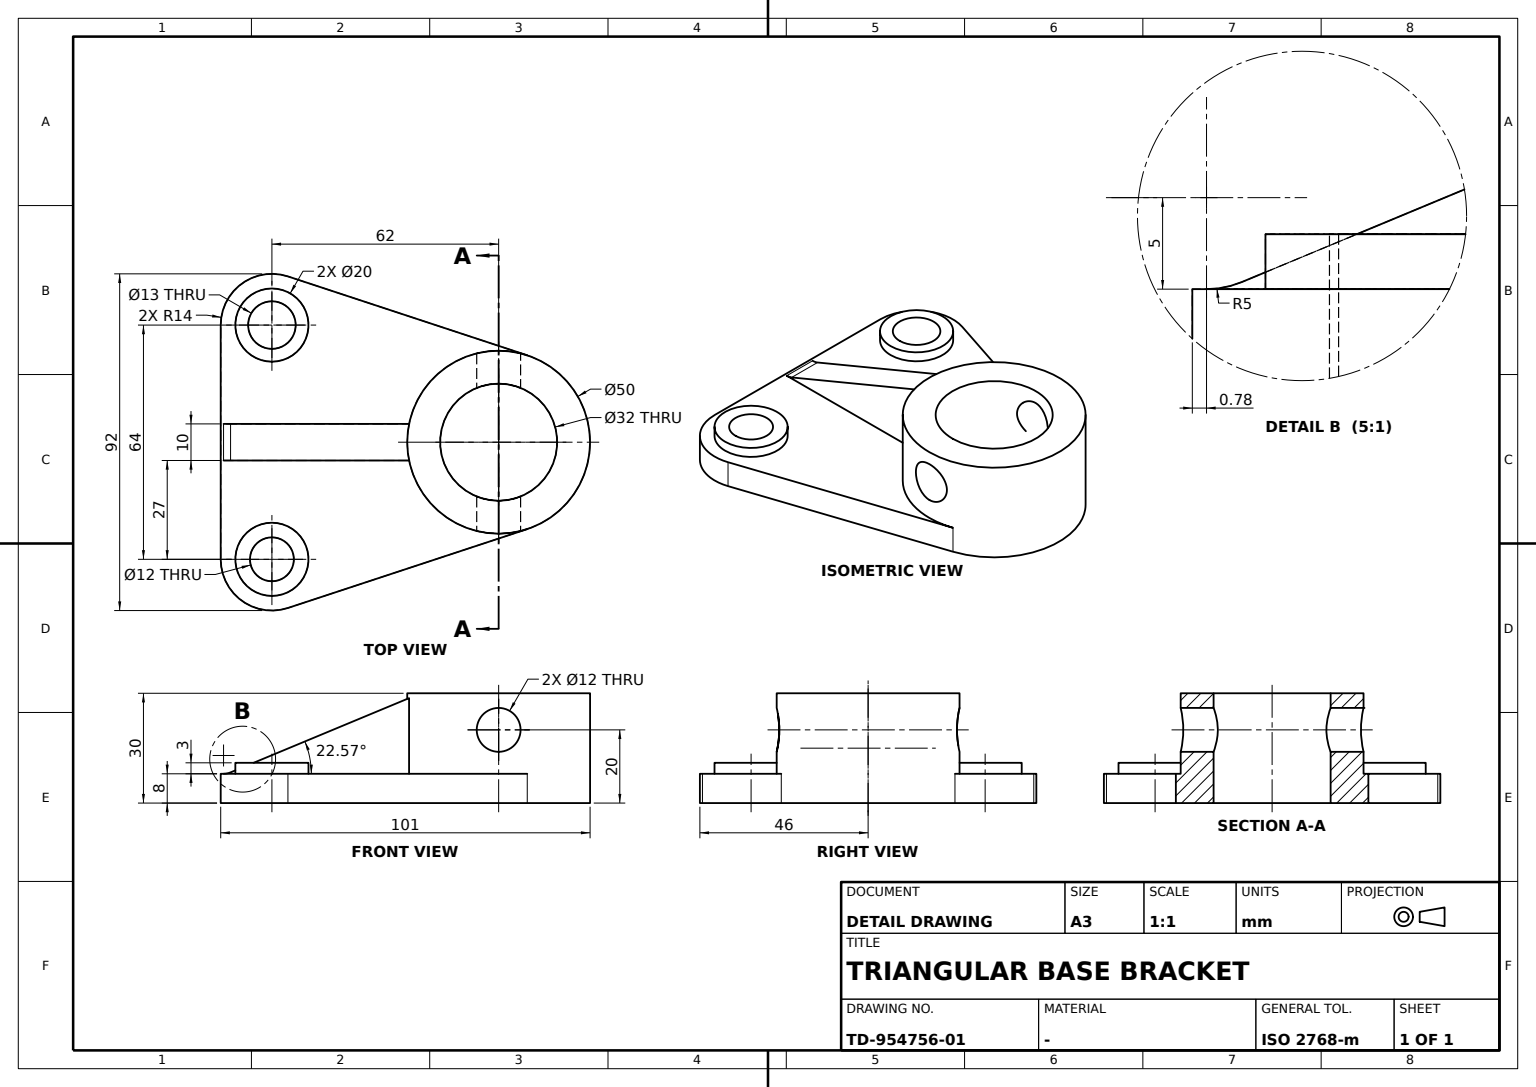
ISO-10303-21;
HEADER;
FILE_DESCRIPTION((''),'2;1');
FILE_NAME('','',(''),(''),'','','');
FILE_SCHEMA(('AUTOMOTIVE_DESIGN'));
ENDSEC;
DATA;
#1=APPLICATION_CONTEXT('');
#2=PRODUCT_CONTEXT('',#1,'mechanical');
#3=PRODUCT('','','',(#2));
#4=PRODUCT_DEFINITION_FORMATION('','',#3);
#5=PRODUCT_DEFINITION_CONTEXT('',#1,'design');
#6=PRODUCT_DEFINITION('','',#4,#5);
#7=PRODUCT_DEFINITION_SHAPE('','',#6);
#8=(LENGTH_UNIT()NAMED_UNIT(*)SI_UNIT(.MILLI.,.METRE.));
#9=(NAMED_UNIT(*)PLANE_ANGLE_UNIT()SI_UNIT($,.RADIAN.));
#10=(NAMED_UNIT(*)SI_UNIT($,.STERADIAN.)SOLID_ANGLE_UNIT());
#11=UNCERTAINTY_MEASURE_WITH_UNIT(LENGTH_MEASURE(0.005),#8,'distance_accuracy_value','');
#12=(GEOMETRIC_REPRESENTATION_CONTEXT(3)GLOBAL_UNCERTAINTY_ASSIGNED_CONTEXT((#11))GLOBAL_UNIT_ASSIGNED_CONTEXT((#8,#9,#10))REPRESENTATION_CONTEXT('',''));
#13=CARTESIAN_POINT('',(5.,-24.494897,8.));
#14=VERTEX_POINT('',#13);
#15=CARTESIAN_POINT('',(5.,-24.494897,28.67148));
#16=VERTEX_POINT('',#15);
#17=DIRECTION('',(0.,0.,1.));
#18=VECTOR('',#17,1000.);
#19=LINE('',#13,#18);
#20=EDGE_CURVE('',#14,#16,#19,.T.);
#21=ORIENTED_EDGE('',*,*,#20,.T.);
#22=CARTESIAN_POINT('',(5.,-73.303678,8.382988));
#23=VERTEX_POINT('',#22);
#24=CARTESIAN_POINT('',(5.,-76.,7.2622));
#25=DIRECTION('',(0.,0.923402354,0.383833418));
#26=VECTOR('',#25,1000.);
#27=LINE('',#24,#26);
#28=EDGE_CURVE('',#23,#16,#27,.T.);
#29=ORIENTED_EDGE('',*,*,#28,.F.);
#30=CARTESIAN_POINT('',(5.,-75.222845,8.));
#31=VERTEX_POINT('',#30);
#32=CARTESIAN_POINT('',(5.,-75.222845,13.));
#33=DIRECTION('',(1.,0.,0.));
#34=DIRECTION('',(0.,0.,-1.));
#35=AXIS2_PLACEMENT_3D('',#32,#33,#34);
#36=CIRCLE('',#35,5.);
#37=EDGE_CURVE('',#31,#23,#36,.T.);
#38=ORIENTED_EDGE('',*,*,#37,.F.);
#39=CARTESIAN_POINT('',(5.,0.,8.));
#40=DIRECTION('',(0.,-1.,0.));
#41=VECTOR('',#40,1000.);
#42=LINE('',#39,#41);
#43=EDGE_CURVE('',#14,#31,#42,.T.);
#44=ORIENTED_EDGE('',*,*,#43,.F.);
#45=EDGE_LOOP('',(#21,#29,#38,#44));
#46=FACE_BOUND('',#45,.T.);
#47=CARTESIAN_POINT('',(5.,0.,0.));
#48=DIRECTION('',(0.,1.,0.));
#49=AXIS2_PLACEMENT_3D('',#47,#33,#48);
#50=PLANE('',#49);
#51=ADVANCED_FACE('',(#46),#50,.T.);
#52=CARTESIAN_POINT('',(-25.5,-62.,0.));
#53=VERTEX_POINT('',#52);
#54=CARTESIAN_POINT('',(-32.,-62.,0.));
#55=AXIS2_PLACEMENT_3D('',#54,#17,#33);
#56=CIRCLE('',#55,6.5);
#57=EDGE_CURVE('',#53,#53,#56,.T.);
#58=ORIENTED_EDGE('',*,*,#57,.T.);
#59=EDGE_LOOP('',(#58));
#60=FACE_BOUND('',#59,.T.);
#61=CARTESIAN_POINT('',(16.,0.,0.));
#62=VERTEX_POINT('',#61);
#63=CARTESIAN_POINT('',(0.,0.,0.));
#64=AXIS2_PLACEMENT_3D('',#63,#17,#33);
#65=CIRCLE('',#64,16.);
#66=EDGE_CURVE('',#62,#62,#65,.T.);
#67=ORIENTED_EDGE('',*,*,#66,.T.);
#68=EDGE_LOOP('',(#67));
#69=FACE_BOUND('',#68,.T.);
#70=CARTESIAN_POINT('',(-45.297428,-57.620683,0.));
#71=VERTEX_POINT('',#70);
#72=CARTESIAN_POINT('',(-32.,-76.,0.));
#73=VERTEX_POINT('',#72);
#74=CIRCLE('',#55,14.);
#75=EDGE_CURVE('',#71,#73,#74,.T.);
#76=ORIENTED_EDGE('',*,*,#75,.F.);
#77=CARTESIAN_POINT('',(-23.745406,7.82021,0.));
#78=VERTEX_POINT('',#77);
#79=DIRECTION('',(-0.312808388,-0.949816252,0.));
#80=VECTOR('',#79,1000.);
#81=LINE('',#77,#80);
#82=EDGE_CURVE('',#78,#71,#81,.T.);
#83=ORIENTED_EDGE('',*,*,#82,.F.);
#84=CARTESIAN_POINT('',(23.745406,7.82021,0.));
#85=VERTEX_POINT('',#84);
#86=CIRCLE('',#64,25.);
#87=EDGE_CURVE('',#85,#78,#86,.T.);
#88=ORIENTED_EDGE('',*,*,#87,.F.);
#89=CARTESIAN_POINT('',(45.297428,-57.620683,0.));
#90=VERTEX_POINT('',#89);
#91=DIRECTION('',(0.312808388,-0.949816252,0.));
#92=VECTOR('',#91,1000.);
#93=LINE('',#84,#92);
#94=EDGE_CURVE('',#85,#90,#93,.T.);
#95=ORIENTED_EDGE('',*,*,#94,.T.);
#96=CARTESIAN_POINT('',(32.,-76.,0.));
#97=VERTEX_POINT('',#96);
#98=CARTESIAN_POINT('',(32.,-62.,0.));
#99=AXIS2_PLACEMENT_3D('',#98,#17,#33);
#100=CIRCLE('',#99,14.);
#101=EDGE_CURVE('',#97,#90,#100,.T.);
#102=ORIENTED_EDGE('',*,*,#101,.F.);
#103=CARTESIAN_POINT('',(0.,-76.,0.));
#104=VECTOR('',#33,1000.);
#105=LINE('',#103,#104);
#106=EDGE_CURVE('',#73,#97,#105,.T.);
#107=ORIENTED_EDGE('',*,*,#106,.F.);
#108=EDGE_LOOP('',(#76,#83,#88,#95,#102,#107));
#109=FACE_BOUND('',#108,.T.);
#110=CARTESIAN_POINT('',(38.,-62.,0.));
#111=VERTEX_POINT('',#110);
#112=CIRCLE('',#99,6.);
#113=EDGE_CURVE('',#111,#111,#112,.T.);
#114=ORIENTED_EDGE('',*,*,#113,.T.);
#115=EDGE_LOOP('',(#114));
#116=FACE_BOUND('',#115,.T.);
#117=PLANE('',#64);
#118=ADVANCED_FACE('',(#60,#69,#109,#116),#117,.F.);
#119=CARTESIAN_POINT('',(-45.297428,-57.620683,8.));
#120=VERTEX_POINT('',#119);
#121=CARTESIAN_POINT('',(-45.297428,-57.620683,4.));
#122=LINE('',#121,#18);
#123=EDGE_CURVE('',#71,#120,#122,.T.);
#124=ORIENTED_EDGE('',*,*,#123,.F.);
#125=ORIENTED_EDGE('',*,*,#75,.T.);
#126=CARTESIAN_POINT('',(-32.,-76.,8.));
#127=VERTEX_POINT('',#126);
#128=CARTESIAN_POINT('',(-32.,-76.,4.));
#129=LINE('',#128,#18);
#130=EDGE_CURVE('',#73,#127,#129,.T.);
#131=ORIENTED_EDGE('',*,*,#130,.T.);
#132=CARTESIAN_POINT('',(-32.,-62.,8.));
#133=AXIS2_PLACEMENT_3D('',#132,#17,#33);
#134=CIRCLE('',#133,14.);
#135=EDGE_CURVE('',#120,#127,#134,.T.);
#136=ORIENTED_EDGE('',*,*,#135,.F.);
#137=EDGE_LOOP('',(#124,#125,#131,#136));
#138=FACE_BOUND('',#137,.T.);
#139=CARTESIAN_POINT('',(-32.,-62.,4.));
#140=AXIS2_PLACEMENT_3D('',#139,#17,#33);
#141=CYLINDRICAL_SURFACE('',#140,14.);
#142=ADVANCED_FACE('',(#138),#141,.T.);
#143=CARTESIAN_POINT('',(-22.,-62.,8.));
#144=VERTEX_POINT('',#143);
#145=CIRCLE('',#133,10.);
#146=EDGE_CURVE('',#144,#144,#145,.T.);
#147=ORIENTED_EDGE('',*,*,#146,.T.);
#148=EDGE_LOOP('',(#147));
#149=FACE_BOUND('',#148,.T.);
#150=CARTESIAN_POINT('',(-22.,-62.,11.));
#151=VERTEX_POINT('',#150);
#152=CARTESIAN_POINT('',(-32.,-62.,11.));
#153=AXIS2_PLACEMENT_3D('',#152,#17,#33);
#154=CIRCLE('',#153,10.);
#155=EDGE_CURVE('',#151,#151,#154,.T.);
#156=ORIENTED_EDGE('',*,*,#155,.F.);
#157=EDGE_LOOP('',(#156));
#158=FACE_BOUND('',#157,.T.);
#159=CARTESIAN_POINT('',(-32.,-62.,9.5));
#160=AXIS2_PLACEMENT_3D('',#159,#17,#33);
#161=CYLINDRICAL_SURFACE('',#160,10.);
#162=ADVANCED_FACE('',(#149,#158),#161,.T.);
#163=CARTESIAN_POINT('',(14.832397,-6.,20.));
#164=VERTEX_POINT('',#163);
#165=CARTESIAN_POINT('',(15.438638,-4.702504,15.296631));
#166=CARTESIAN_POINT('',(14.529476,-6.648414,20.000931));
#167=CARTESIAN_POINT('',(15.437841,-4.703839,24.699646));
#168=CARTESIAN_POINT('',(16.281291,0.002975,26.651377));
#169=CARTESIAN_POINT('',(15.436993,4.705057,24.694845));
#170=CARTESIAN_POINT('',(14.529843,6.648585,20.009134));
#171=CARTESIAN_POINT('',(15.43802,4.700591,15.296493));
#172=CARTESIAN_POINT('',(16.280835,0.007567,13.351722));
#173=B_SPLINE_CURVE_WITH_KNOTS('',3,(#165,#166,#167,#168,#169,#170,#171,#172,#165,#166,#167),.UNSPECIFIED.,.T.,.F.,(1,1,1,1,1,1,1,1,1,1,1,1,1,1,1),(-0.014193849,-0.009462566,-0.004731283,0.,0.004731283,0.009462566,0.014193849,0.018925132,0.023656415,0.028387698,0.033118981,0.037850264,0.042581547,0.04731283,0.052044113),.UNSPECIFIED.);
#174=EDGE_CURVE('',#164,#164,#173,.T.);
#175=ORIENTED_EDGE('',*,*,#174,.T.);
#176=EDGE_LOOP('',(#175));
#177=FACE_BOUND('',#176,.T.);
#178=CARTESIAN_POINT('',(25.,0.,14.));
#179=VERTEX_POINT('',#178);
#180=CARTESIAN_POINT('',(24.640168,-4.700584,24.702732));
#181=CARTESIAN_POINT('',(24.083983,-6.649013,19.99808));
#182=CARTESIAN_POINT('',(24.639835,-4.703363,15.300168));
#183=CARTESIAN_POINT('',(25.179986,0.001317,13.350708));
#184=CARTESIAN_POINT('',(24.640221,4.700485,15.297001));
#185=CARTESIAN_POINT('',(24.083956,6.649063,20.00192));
#186=CARTESIAN_POINT('',(24.639887,4.703263,24.7001));
#187=CARTESIAN_POINT('',(25.179986,-0.002041,26.649292));
#188=B_SPLINE_CURVE_WITH_KNOTS('',3,(#180,#181,#182,#183,#184,#185,#186,#187,#180,#181,#182),.UNSPECIFIED.,.T.,.F.,(1,1,1,1,1,1,1,1,1,1,1,1,1,1,1),(0.004704535,0.009408284,0.014112033,0.018815782,0.023519531,0.02822328,0.032927029,0.037630779,0.042334528,0.047038277,0.051742026,0.056445775,0.061149524,0.065853273,0.070557022),.UNSPECIFIED.);
#189=EDGE_CURVE('',#179,#179,#188,.T.);
#190=ORIENTED_EDGE('',*,*,#189,.T.);
#191=EDGE_LOOP('',(#190));
#192=FACE_BOUND('',#191,.T.);
#193=CARTESIAN_POINT('',(23.66,0.,20.));
#194=AXIS2_PLACEMENT_3D('',#193,#33,#48);
#195=CYLINDRICAL_SURFACE('',#194,6.);
#196=ADVANCED_FACE('',(#177,#192),#195,.F.);
#197=CARTESIAN_POINT('',(-5.,-73.303678,8.382988));
#198=VERTEX_POINT('',#197);
#199=CARTESIAN_POINT('',(0.,-73.303678,8.382988));
#200=LINE('',#199,#104);
#201=EDGE_CURVE('',#198,#23,#200,.T.);
#202=ORIENTED_EDGE('',*,*,#201,.F.);
#203=CARTESIAN_POINT('',(-5.,-75.222845,8.));
#204=VERTEX_POINT('',#203);
#205=CARTESIAN_POINT('',(-5.,-75.222845,13.));
#206=AXIS2_PLACEMENT_3D('',#205,#33,#34);
#207=CIRCLE('',#206,5.);
#208=EDGE_CURVE('',#204,#198,#207,.T.);
#209=ORIENTED_EDGE('',*,*,#208,.F.);
#210=CARTESIAN_POINT('',(0.,-75.222845,8.));
#211=LINE('',#210,#104);
#212=EDGE_CURVE('',#204,#31,#211,.T.);
#213=ORIENTED_EDGE('',*,*,#212,.T.);
#214=ORIENTED_EDGE('',*,*,#37,.T.);
#215=EDGE_LOOP('',(#202,#209,#213,#214));
#216=FACE_BOUND('',#215,.T.);
#217=CARTESIAN_POINT('',(0.,-75.222845,13.));
#218=DIRECTION('',(0.,0.383833418,-0.923402354));
#219=AXIS2_PLACEMENT_3D('',#217,#33,#218);
#220=CYLINDRICAL_SURFACE('',#219,5.);
#221=ADVANCED_FACE('',(#216),#220,.F.);
#222=CARTESIAN_POINT('',(42.,-62.,8.));
#223=VERTEX_POINT('',#222);
#224=CARTESIAN_POINT('',(32.,-62.,8.));
#225=AXIS2_PLACEMENT_3D('',#224,#17,#33);
#226=CIRCLE('',#225,10.);
#227=EDGE_CURVE('',#223,#223,#226,.T.);
#228=ORIENTED_EDGE('',*,*,#227,.T.);
#229=EDGE_LOOP('',(#228));
#230=FACE_BOUND('',#229,.T.);
#231=CARTESIAN_POINT('',(42.,-62.,11.));
#232=VERTEX_POINT('',#231);
#233=CARTESIAN_POINT('',(32.,-62.,11.));
#234=AXIS2_PLACEMENT_3D('',#233,#17,#33);
#235=CIRCLE('',#234,10.);
#236=EDGE_CURVE('',#232,#232,#235,.T.);
#237=ORIENTED_EDGE('',*,*,#236,.F.);
#238=EDGE_LOOP('',(#237));
#239=FACE_BOUND('',#238,.T.);
#240=CARTESIAN_POINT('',(32.,-62.,9.5));
#241=AXIS2_PLACEMENT_3D('',#240,#17,#33);
#242=CYLINDRICAL_SURFACE('',#241,10.);
#243=ADVANCED_FACE('',(#230,#239),#242,.T.);
#244=CARTESIAN_POINT('',(32.,-76.,8.));
#245=VERTEX_POINT('',#244);
#246=CARTESIAN_POINT('',(45.297428,-57.620683,8.));
#247=VERTEX_POINT('',#246);
#248=CIRCLE('',#225,14.);
#249=EDGE_CURVE('',#245,#247,#248,.T.);
#250=ORIENTED_EDGE('',*,*,#249,.F.);
#251=CARTESIAN_POINT('',(32.,-76.,4.));
#252=LINE('',#251,#18);
#253=EDGE_CURVE('',#97,#245,#252,.T.);
#254=ORIENTED_EDGE('',*,*,#253,.F.);
#255=ORIENTED_EDGE('',*,*,#101,.T.);
#256=CARTESIAN_POINT('',(45.297428,-57.620683,4.));
#257=LINE('',#256,#18);
#258=EDGE_CURVE('',#90,#247,#257,.T.);
#259=ORIENTED_EDGE('',*,*,#258,.T.);
#260=EDGE_LOOP('',(#250,#254,#255,#259));
#261=FACE_BOUND('',#260,.T.);
#262=CARTESIAN_POINT('',(32.,-62.,4.));
#263=AXIS2_PLACEMENT_3D('',#262,#17,#33);
#264=CYLINDRICAL_SURFACE('',#263,14.);
#265=ADVANCED_FACE('',(#261),#264,.T.);
#266=CARTESIAN_POINT('',(-25.5,-62.,11.));
#267=VERTEX_POINT('',#266);
#268=CIRCLE('',#153,6.5);
#269=EDGE_CURVE('',#267,#267,#268,.T.);
#270=ORIENTED_EDGE('',*,*,#269,.F.);
#271=EDGE_LOOP('',(#270));
#272=FACE_BOUND('',#271,.T.);
#273=ORIENTED_EDGE('',*,*,#155,.T.);
#274=EDGE_LOOP('',(#273));
#275=FACE_BOUND('',#274,.T.);
#276=CARTESIAN_POINT('',(0.,0.,11.));
#277=AXIS2_PLACEMENT_3D('',#276,#17,#33);
#278=PLANE('',#277);
#279=ADVANCED_FACE('',(#272,#275),#278,.T.);
#280=ORIENTED_EDGE('',*,*,#227,.F.);
#281=EDGE_LOOP('',(#280));
#282=FACE_BOUND('',#281,.T.);
#283=ORIENTED_EDGE('',*,*,#43,.T.);
#284=ORIENTED_EDGE('',*,*,#212,.F.);
#285=CARTESIAN_POINT('',(-5.,-24.494897,8.));
#286=VERTEX_POINT('',#285);
#287=CARTESIAN_POINT('',(-5.,0.,8.));
#288=LINE('',#287,#41);
#289=EDGE_CURVE('',#286,#204,#288,.T.);
#290=ORIENTED_EDGE('',*,*,#289,.F.);
#291=CARTESIAN_POINT('',(-23.745406,7.82021,8.));
#292=VERTEX_POINT('',#291);
#293=CARTESIAN_POINT('',(0.,0.,8.));
#294=AXIS2_PLACEMENT_3D('',#293,#17,#33);
#295=CIRCLE('',#294,25.);
#296=EDGE_CURVE('',#292,#286,#295,.T.);
#297=ORIENTED_EDGE('',*,*,#296,.F.);
#298=LINE('',#291,#80);
#299=EDGE_CURVE('',#292,#120,#298,.T.);
#300=ORIENTED_EDGE('',*,*,#299,.T.);
#301=ORIENTED_EDGE('',*,*,#135,.T.);
#302=CARTESIAN_POINT('',(0.,-76.,8.));
#303=LINE('',#302,#104);
#304=EDGE_CURVE('',#127,#245,#303,.T.);
#305=ORIENTED_EDGE('',*,*,#304,.T.);
#306=ORIENTED_EDGE('',*,*,#249,.T.);
#307=CARTESIAN_POINT('',(23.745406,7.82021,8.));
#308=VERTEX_POINT('',#307);
#309=LINE('',#307,#92);
#310=EDGE_CURVE('',#308,#247,#309,.T.);
#311=ORIENTED_EDGE('',*,*,#310,.F.);
#312=EDGE_CURVE('',#14,#308,#295,.T.);
#313=ORIENTED_EDGE('',*,*,#312,.F.);
#314=EDGE_LOOP('',(#283,#284,#290,#297,#300,#301,#305,#306,#311,#313));
#315=FACE_BOUND('',#314,.T.);
#316=ORIENTED_EDGE('',*,*,#146,.F.);
#317=EDGE_LOOP('',(#316));
#318=FACE_BOUND('',#317,.T.);
#319=PLANE('',#294);
#320=ADVANCED_FACE('',(#282,#315,#318),#319,.T.);
#321=CARTESIAN_POINT('',(-14.832397,6.,20.));
#322=VERTEX_POINT('',#321);
#323=CARTESIAN_POINT('',(-15.43811,-4.702049,24.701313));
#324=CARTESIAN_POINT('',(-14.529709,-6.648345,19.999768));
#325=CARTESIAN_POINT('',(-15.437434,-4.704571,15.301256));
#326=CARTESIAN_POINT('',(-16.281119,0.000146,13.350008));
#327=CARTESIAN_POINT('',(-15.438088,4.702119,15.298712));
#328=CARTESIAN_POINT('',(-14.529709,6.648345,20.000424));
#329=CARTESIAN_POINT('',(-15.437456,4.704501,24.69877));
#330=CARTESIAN_POINT('',(-16.281108,-0.000146,26.649979));
#331=B_SPLINE_CURVE_WITH_KNOTS('',3,(#323,#324,#325,#326,#327,#328,#329,#330,#323,#324,#325),.UNSPECIFIED.,.T.,.F.,(1,1,1,1,1,1,1,1,1,1,1,1,1,1,1),(-0.014190832,-0.009460645,-0.004730457,-0.000000269,0.004729918,0.009460106,0.014190293,0.018920481,0.023650668,0.028380856,0.033111044,0.037841231,0.042571419,0.047301606,0.052031794),.UNSPECIFIED.);
#332=EDGE_CURVE('',#322,#322,#331,.T.);
#333=ORIENTED_EDGE('',*,*,#332,.T.);
#334=EDGE_LOOP('',(#333));
#335=FACE_BOUND('',#334,.T.);
#336=CARTESIAN_POINT('',(-25.,0.,26.));
#337=VERTEX_POINT('',#336);
#338=CARTESIAN_POINT('',(-24.640168,-4.700584,15.297268));
#339=CARTESIAN_POINT('',(-24.083983,-6.649013,20.00192));
#340=CARTESIAN_POINT('',(-24.639835,-4.703363,24.699832));
#341=CARTESIAN_POINT('',(-25.179986,0.001317,26.649292));
#342=CARTESIAN_POINT('',(-24.640221,4.700485,24.702999));
#343=CARTESIAN_POINT('',(-24.083956,6.649063,19.99808));
#344=CARTESIAN_POINT('',(-24.639887,4.703263,15.2999));
#345=CARTESIAN_POINT('',(-25.179986,-0.002041,13.350708));
#346=B_SPLINE_CURVE_WITH_KNOTS('',3,(#338,#339,#340,#341,#342,#343,#344,#345,#338,#339,#340),.UNSPECIFIED.,.T.,.F.,(1,1,1,1,1,1,1,1,1,1,1,1,1,1,1),(0.004704535,0.009408284,0.014112033,0.018815782,0.023519531,0.02822328,0.032927029,0.037630779,0.042334528,0.047038277,0.051742026,0.056445775,0.061149524,0.065853273,0.070557022),.UNSPECIFIED.);
#347=EDGE_CURVE('',#337,#337,#346,.T.);
#348=ORIENTED_EDGE('',*,*,#347,.T.);
#349=EDGE_LOOP('',(#348));
#350=FACE_BOUND('',#349,.T.);
#351=ADVANCED_FACE('',(#335,#350),#195,.F.);
#352=ORIENTED_EDGE('',*,*,#20,.F.);
#353=ORIENTED_EDGE('',*,*,#312,.T.);
#354=CARTESIAN_POINT('',(23.745406,7.82021,19.));
#355=LINE('',#354,#18);
#356=EDGE_CURVE('',#85,#308,#355,.T.);
#357=ORIENTED_EDGE('',*,*,#356,.F.);
#358=ORIENTED_EDGE('',*,*,#87,.T.);
#359=CARTESIAN_POINT('',(-23.745406,7.82021,19.));
#360=LINE('',#359,#18);
#361=EDGE_CURVE('',#78,#292,#360,.T.);
#362=ORIENTED_EDGE('',*,*,#361,.T.);
#363=ORIENTED_EDGE('',*,*,#296,.T.);
#364=CARTESIAN_POINT('',(-5.,-24.494897,28.67148));
#365=VERTEX_POINT('',#364);
#366=LINE('',#285,#18);
#367=EDGE_CURVE('',#286,#365,#366,.T.);
#368=ORIENTED_EDGE('',*,*,#367,.T.);
#369=CARTESIAN_POINT('',(0.,0.,38.853347));
#370=DIRECTION('',(0.,-0.383833418,0.923402354));
#371=AXIS2_PLACEMENT_3D('',#369,#370,#25);
#372=ELLIPSE('',#371,27.073788,25.);
#373=EDGE_CURVE('',#365,#16,#372,.T.);
#374=ORIENTED_EDGE('',*,*,#373,.T.);
#375=EDGE_LOOP('',(#352,#353,#357,#358,#362,#363,#368,#374));
#376=FACE_BOUND('',#375,.T.);
#377=CARTESIAN_POINT('',(25.,0.,30.));
#378=VERTEX_POINT('',#377);
#379=CARTESIAN_POINT('',(0.,0.,30.));
#380=AXIS2_PLACEMENT_3D('',#379,#17,#33);
#381=CIRCLE('',#380,25.);
#382=EDGE_CURVE('',#378,#378,#381,.T.);
#383=ORIENTED_EDGE('',*,*,#382,.F.);
#384=EDGE_LOOP('',(#383));
#385=FACE_BOUND('',#384,.T.);
#386=ORIENTED_EDGE('',*,*,#347,.F.);
#387=EDGE_LOOP('',(#386));
#388=FACE_BOUND('',#387,.T.);
#389=ORIENTED_EDGE('',*,*,#189,.F.);
#390=EDGE_LOOP('',(#389));
#391=FACE_BOUND('',#390,.T.);
#392=CARTESIAN_POINT('',(0.,0.,19.));
#393=AXIS2_PLACEMENT_3D('',#392,#17,#33);
#394=CYLINDRICAL_SURFACE('',#393,25.);
#395=ADVANCED_FACE('',(#376,#385,#388,#391),#394,.T.);
#396=ORIENTED_EDGE('',*,*,#332,.F.);
#397=EDGE_LOOP('',(#396));
#398=FACE_BOUND('',#397,.T.);
#399=ORIENTED_EDGE('',*,*,#174,.F.);
#400=EDGE_LOOP('',(#399));
#401=FACE_BOUND('',#400,.T.);
#402=CARTESIAN_POINT('',(16.,0.,30.));
#403=VERTEX_POINT('',#402);
#404=CIRCLE('',#380,16.);
#405=EDGE_CURVE('',#403,#403,#404,.T.);
#406=ORIENTED_EDGE('',*,*,#405,.T.);
#407=EDGE_LOOP('',(#406));
#408=FACE_BOUND('',#407,.T.);
#409=ORIENTED_EDGE('',*,*,#66,.F.);
#410=EDGE_LOOP('',(#409));
#411=FACE_BOUND('',#410,.T.);
#412=CYLINDRICAL_SURFACE('',#393,16.);
#413=ADVANCED_FACE('',(#398,#401,#408,#411),#412,.F.);
#414=ORIENTED_EDGE('',*,*,#82,.T.);
#415=ORIENTED_EDGE('',*,*,#123,.T.);
#416=ORIENTED_EDGE('',*,*,#299,.F.);
#417=ORIENTED_EDGE('',*,*,#361,.F.);
#418=EDGE_LOOP('',(#414,#415,#416,#417));
#419=FACE_BOUND('',#418,.T.);
#420=DIRECTION('',(-0.949816252,0.312808388,0.));
#421=AXIS2_PLACEMENT_3D('',#77,#420,#79);
#422=PLANE('',#421);
#423=ADVANCED_FACE('',(#419),#422,.T.);
#424=ORIENTED_EDGE('',*,*,#258,.F.);
#425=ORIENTED_EDGE('',*,*,#94,.F.);
#426=ORIENTED_EDGE('',*,*,#356,.T.);
#427=ORIENTED_EDGE('',*,*,#310,.T.);
#428=EDGE_LOOP('',(#424,#425,#426,#427));
#429=FACE_BOUND('',#428,.T.);
#430=DIRECTION('',(-0.949816252,-0.312808388,0.));
#431=AXIS2_PLACEMENT_3D('',#84,#430,#91);
#432=PLANE('',#431);
#433=ADVANCED_FACE('',(#429),#432,.F.);
#434=ORIENTED_EDGE('',*,*,#201,.T.);
#435=ORIENTED_EDGE('',*,*,#28,.T.);
#436=ORIENTED_EDGE('',*,*,#373,.F.);
#437=CARTESIAN_POINT('',(-5.,-76.,7.2622));
#438=LINE('',#437,#26);
#439=EDGE_CURVE('',#198,#365,#438,.T.);
#440=ORIENTED_EDGE('',*,*,#439,.F.);
#441=EDGE_LOOP('',(#434,#435,#436,#440));
#442=FACE_BOUND('',#441,.T.);
#443=CARTESIAN_POINT('',(0.,-76.,7.2622));
#444=DIRECTION('',(0.,-0.923402354,-0.383833418));
#445=AXIS2_PLACEMENT_3D('',#443,#370,#444);
#446=PLANE('',#445);
#447=ADVANCED_FACE('',(#442),#446,.T.);
#448=ORIENTED_EDGE('',*,*,#236,.T.);
#449=EDGE_LOOP('',(#448));
#450=FACE_BOUND('',#449,.T.);
#451=CARTESIAN_POINT('',(38.,-62.,11.));
#452=VERTEX_POINT('',#451);
#453=CIRCLE('',#234,6.);
#454=EDGE_CURVE('',#452,#452,#453,.T.);
#455=ORIENTED_EDGE('',*,*,#454,.F.);
#456=EDGE_LOOP('',(#455));
#457=FACE_BOUND('',#456,.T.);
#458=ADVANCED_FACE('',(#450,#457),#278,.T.);
#459=ORIENTED_EDGE('',*,*,#57,.F.);
#460=EDGE_LOOP('',(#459));
#461=FACE_BOUND('',#460,.T.);
#462=ORIENTED_EDGE('',*,*,#269,.T.);
#463=EDGE_LOOP('',(#462));
#464=FACE_BOUND('',#463,.T.);
#465=CYLINDRICAL_SURFACE('',#160,6.5);
#466=ADVANCED_FACE('',(#461,#464),#465,.F.);
#467=ORIENTED_EDGE('',*,*,#454,.T.);
#468=EDGE_LOOP('',(#467));
#469=FACE_BOUND('',#468,.T.);
#470=ORIENTED_EDGE('',*,*,#113,.F.);
#471=EDGE_LOOP('',(#470));
#472=FACE_BOUND('',#471,.T.);
#473=CYLINDRICAL_SURFACE('',#241,6.);
#474=ADVANCED_FACE('',(#469,#472),#473,.F.);
#475=ORIENTED_EDGE('',*,*,#304,.F.);
#476=ORIENTED_EDGE('',*,*,#130,.F.);
#477=ORIENTED_EDGE('',*,*,#106,.T.);
#478=ORIENTED_EDGE('',*,*,#253,.T.);
#479=EDGE_LOOP('',(#475,#476,#477,#478));
#480=FACE_BOUND('',#479,.T.);
#481=AXIS2_PLACEMENT_3D('',#72,#40,#33);
#482=PLANE('',#481);
#483=ADVANCED_FACE('',(#480),#482,.T.);
#484=ORIENTED_EDGE('',*,*,#289,.T.);
#485=ORIENTED_EDGE('',*,*,#208,.T.);
#486=ORIENTED_EDGE('',*,*,#439,.T.);
#487=ORIENTED_EDGE('',*,*,#367,.F.);
#488=EDGE_LOOP('',(#484,#485,#486,#487));
#489=FACE_BOUND('',#488,.T.);
#490=CARTESIAN_POINT('',(-5.,0.,0.));
#491=AXIS2_PLACEMENT_3D('',#490,#33,#48);
#492=PLANE('',#491);
#493=ADVANCED_FACE('',(#489),#492,.F.);
#494=ORIENTED_EDGE('',*,*,#382,.T.);
#495=EDGE_LOOP('',(#494));
#496=FACE_BOUND('',#495,.T.);
#497=ORIENTED_EDGE('',*,*,#405,.F.);
#498=EDGE_LOOP('',(#497));
#499=FACE_BOUND('',#498,.T.);
#500=PLANE('',#380);
#501=ADVANCED_FACE('',(#496,#499),#500,.T.);
#502=CLOSED_SHELL('',(#51,#118,#142,#162,#196,#221,#243,#265,#279,#320,#351,#395,#413,#423,#433,#447,#458,#466,#474,#483,#493,#501));
#503=MANIFOLD_SOLID_BREP('',#502);
#504=ADVANCED_BREP_SHAPE_REPRESENTATION('',(#503),#12);
#505=SHAPE_DEFINITION_REPRESENTATION(#7,#504);
ENDSEC;
END-ISO-10303-21;
